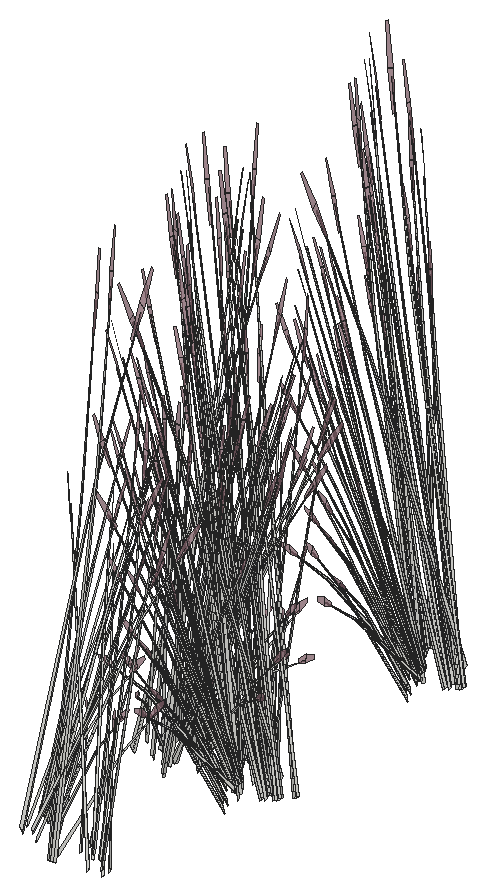
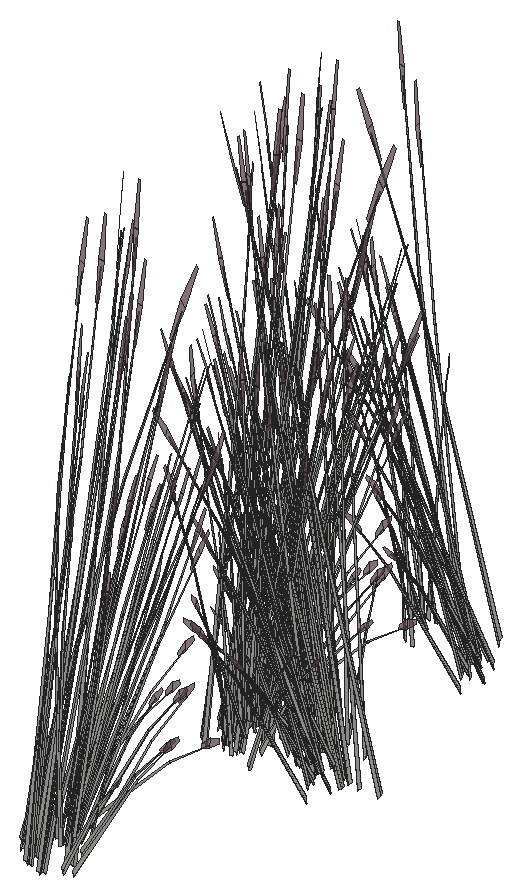
# SketchUp Ruby script. Lengths in inches.
U = 1.inch
M = Sketchup.active_model
def pt(a) = Geom::Point3d.new(a.map { |v| v * U })
def face(e, loops, mat)
  f = e.add_face(loops[0].map { |a| pt(a) })
  loops[1..].each { |l| e.add_face(l.map { |a| pt(a) }).erase! }
  f.material = f.back_material = mat if mat
  f
end
# faces: each face lists its corners as indices into pts; further lists are holes
def faces(e, pts, list, mat = nil) = list.each { |f| face(e, (f[0].is_a?(Array) ? f : [f]).map { |l| l.map { |i| pts[i] } }, mat) }
# xy, xz, yz: faces in a plane at the given z, y or x. An outline is a flat list of corners, or four numbers for a rectangle; further outlines are holes
def ring(l) = l.size == 4 ? [[l[0], l[1]], [l[2], l[1]], [l[2], l[3]], [l[0], l[3]]] : l.each_slice(2).to_a
def flat(e, list, mat, &to3) = list.each { |f| face(e, (f[0].is_a?(Array) ? f : [f]).map { |l| ring(l).map { |u, v| to3.(u, v) } }, mat) }
def xy(e, z, list, mat = nil) = flat(e, list, mat) { |x, y| [x, y, z] }
def xz(e, y, list, mat = nil) = flat(e, list, mat) { |x, z| [x, y, z] }
def yz(e, x, list, mat = nil) = flat(e, list, mat) { |y, z| [x, y, z] }
def lines(e, pts, list) = list.each { |a, b| e.add_line(pt(pts[a]), pt(pts[b])) }
# prism: a flat outline (further loops are holes) pulled along v
def prism(e, loops, v, mat = nil)
  f = face(e, loops, mat); d = Geom::Vector3d.new(v.map { |x| x * U })
  f.pushpull(f.normal.samedirection?(d) ? d.length : -d.length)
end
def box(e, o, s, mat = nil) = prism(e, [[o, [o[0] + s[0], o[1], o[2]], [o[0] + s[0], o[1] + s[1], o[2]], [o[0], o[1] + s[1], o[2]]]], [0, 0, s[2]], mat)
def at(x, y, z, deg = 0) = Geom::Transformation.translation(pt([x, y, z])) * Geom::Transformation.rotation(ORIGIN, Z_AXIS, deg.degrees)
def axes(o, x, y, z) = Geom::Transformation.new([*x, 0, *y, 0, *z, 0, *pt(o).to_a, 1])
def part(name) = M.definitions.add(name)
# library, detail: a bought-in or finely detailed component or shape, given as its bounding box
def library(name, o, s) = part(name).tap { |d| box(d.entities, o, s) }
def detail(e, o, s) = box(e.add_group.entities, o, s)
def put(e, d, t, mat = nil) = e.add_instance(d, t).tap { |i| i.material = mat if mat }
def group(e, t, mat = nil) = e.add_group.tap { |g| g.transformation = t; g.material = mat if mat }.entities
root = M.entities
M.materials.add("LightPink_Translucent").color = [144, 107, 117]
M.materials["LightPink_Translucent"].alpha = 0.75
c1 = part("blade")
p = [[2.15,0.21,22],[0,0.17,0],[0.09,0.45,0],[2.18,0.31,22],[2.29,0.31,22],[0.38,0.45,0],
  [2.48,0.24,33],[2.49,0.24,33],[2.48,0.22,33]]
faces(c1.entities,p,[[0,1,2,3],[4,5,2,3],[6,3,4,7],[8,0,3,6]])
c2 = part("seeds")
p = [[0.3,-0.1,1.38],[-0.01,-0.03,1.59],[-0.01,-0.03,0.03],[0.14,-0.07,-0.07],[0.29,-0.03,3],[0.15,0.01,3.11]]
faces(c2.entities,p,[[0,1,2,3],[1,0,4,5]],"LightPink_Translucent")
c3 = part("blade with seeds")
put(c3.entities,c1,at(0,0,0))
put(c3.entities,c2,axes([2.4,0.25,30.99],[1.5799,-0.05474,1.17369],[-0.12525,1.92788,0.29478],[-0.07173,-0.02425,1.56792]))
put(root,c3,axes([503.59,165.17,3.07],[0.14147,-0.21002,1.71376],[0.59349,0.43464,0.13857],[-0.26773,0.27089,0.73262]))
put(root,c3,axes([498.37,167.02,1.57],[0.95008,0,0],[0,0.68292,-0.51607],[0,0.15554,1.63711]))
put(root,c3,axes([503.76,166.35,3.72],[-0.5141,0.32171,-0.35414],[-0.48666,-0.36734,0.4572],[-0.07405,0.18664,0.87481]))
put(root,c3,axes([501.98,166.26,3.91],[-0.01889,0.12092,1.74944],[0.53598,0.42065,-0.27667],[-0.14032,0.19892,0.14031]))
put(root,c3,axes([497.58,168.53,3.72],[0.43232,0.38257,-0.35414],[-0.49364,0.36215,0.4572],[0.25081,0.0551,0.87481]))
put(root,c3,axes([497.36,168.68,3.92],[-0.03826,0.46465,0.0643],[-0.57772,-0.01274,0.50621],[0.2213,0.04862,0.77189]))
put(root,c3,axes([504.08,167.6,1.96],[-0.01966,-0.36332,1.1486],[0.49135,0.25914,0.84392],[-0.09663,0.17317,0.25299]))
put(root,c3,axes([497.42,168.53,3.93],[-0.56024,0.40262,0.48003],[-0.48318,-0.42758,0.3958],[0.26285,0.07427,0.9933]))
put(root,c3,axes([504.27,166.2,4.2],[0.54391,0.41056,-0.5672],[-0.57458,0.35956,-0.43934],[-0.08276,0.2086,1.08528]))
put(root,c3,axes([495.63,168.99,4.24],[-0.11735,-0.49217,0.35414],[0.67083,-0.12996,-0.4572],[0.18018,0.14104,0.87481]))
put(root,c3,axes([498.16,167.48,1.21],[0,0.61104,-0.49651],[-0.85008,0,0],[0,0.13917,1.57504]))
put(root,c3,axes([496.03,167.55,3.07],[-0.28223,-0.10528,1.71376],[0.58406,-0.44165,0.13857],[0.36402,0.19924,0.73262]))
put(root,c3,axes([496.08,166.16,3.67],[-0.65655,-0.31748,1.38283],[0.69326,-0.49431,0.59665],[0.21183,0.29789,1.33663]))
put(root,c3,axes([504.1,166.01,4.53],[-0.01977,0.56521,-0.7886],[-0.83252,-0.03796,0.09517],[-0.08786,0.23945,1.11556]))
put(root,c3,axes([501.92,167.5,3.9],[0.0862,-0.03689,1.77383],[0.71245,0.24539,-0.16761],[-0.01674,0.20431,0.31391]))
put(root,c3,axes([497.08,168.75,1.96],[-0.4278,-0.1757,1.1486],[0.5524,-0.17852,0.84392],[0.14899,0.15122,0.25299]))
put(root,c3,axes([495.57,169.25,4.23],[0.45276,-0.52302,-0.1216],[0.65568,0.30132,-0.67495],[0.22792,0.14777,1.02557]))
put(root,c3,axes([494.98,169.68,3.9],[0.00225,-0.07398,1.77383],[0.65113,-0.32638,-0.16761],[0.22617,0.1165,0.31391]))
put(root,c3,axes([497.2,169.4,0.6875],[0.05536,-0.08822,1.76342],[0.69692,-0.25981,-0.26939],[0.21129,0.13447,0.30037]))
put(root,c3,axes([496.11,168.99,3.875],[0.74975,-0.14525,-0.51099],[0.13115,0.55007,-0.3958],[0.20138,0.15763,0.97773]))
put(root,c3,axes([503.51,167.28,1.78],[0.23977,-0.09639,1.43002],[0.59198,0.29065,-0.30754],[-0.1762,0.25149,0.61141]))
put(root,c3,axes([497.14,169.55,1.86],[-0.48723,-0.01916,1.0506],[0.32177,-0.40701,0.58006],[0.19248,0.1446,0.8241]))
put(root,c3,axes([495.74,169.44,3.92],[-0.34533,0.38816,0.0643],[-0.49176,-0.22599,0.50621],[0.15898,0.12445,0.77189]))
put(root,c3,axes([495.89,169.33,3.93],[-0.75571,0.14023,0.48003],[-0.13115,-0.55007,0.3958],[0.17773,0.16212,0.9933]))
put(root,c3,axes([503.82,166.81,2.56],[0.01669,-0.31544,1.54345],[0.75083,0.16661,0.21329],[-0.06506,0.33618,0.72882]))
put(root,c3,axes([495.55,168.5625,1.78],[0.01341,-0.20255,1.43002],[0.64074,-0.22625,-0.30754],[0.1978,0.24243,0.61141]))
put(root,c3,axes([494.87,168.16,3.07],[-0.17368,-0.19618,1.71376],[0.80256,-0.16516,0.13857],[0.18139,0.30799,0.73262]))
put(root,c3,axes([504.63,183.77,3.07],[0.17368,0.19618,1.71376],[-0.80256,0.16516,0.13857],[-0.18139,-0.30799,0.73262]))
put(root,c3,axes([505.96,182.47,3.91],[-0.11621,-0.08567,1.74944],[-0.77555,0.05431,-0.27667],[-0.12378,-0.20491,0.14031]))
put(root,c3,axes([504.41,183.25,1.78],[-0.04601,0.19989,1.43002],[-0.67263,0.16733,-0.30754],[-0.15723,-0.25836,0.61141]))
put(root,c3,axes([505.16,182.1875,3.9],[-0.01417,0.07324,1.77383],[-0.6991,0.2658,-0.16761],[-0.20573,-0.13587,0.31391]))
put(root,c3,axes([505.01,183.49,4.29],[0.84639,-0.15705,0.53763],[0.14689,0.61608,0.4433],[-0.19906,-0.18157,1.11249]))
put(root,c3,axes([504.18,182.93,1.96],[0.39634,0.21267,1.1486],[-0.57721,0.12784,0.84392],[-0.1235,-0.16344,0.25299]))
put(root,c3,axes([505.14,184.06,4.17],[-0.64788,-0.29534,-0.71045],[0.46044,-0.51755,0.08574],[-0.23473,-0.17635,1.00501]))
put(root,c3,axes([504.91,183.66,3.72],[-0.11735,-0.49217,-0.35414],[0.67083,-0.12996,0.4572],[-0.18018,-0.14104,0.87481]))
put(root,c3,axes([505.2,183.62,3.92],[0.34533,-0.38816,0.0643],[0.49176,0.22599,0.50621],[-0.15898,-0.12445,0.77189]))
put(root,c3,axes([503.87,183.57,0.6875],[-0.0736,0.08049,1.76342],[-0.74378,0.17355,-0.26939],[-0.17968,-0.15788,0.30037]))
put(root,c3,axes([496.22,185,3.91],[-0.00733,-0.12161,1.74944],[-0.61946,-0.35147,-0.27667],[0.09577,-0.21306,0.14031]))
put(root,c3,axes([494.12,185.6,3.07],[-0.14147,0.21002,1.71376],[-0.59349,-0.43464,0.13857],[0.26773,-0.27089,0.73262]))
put(root,c3,axes([504.83,184.07,3.875],[-0.74975,0.14525,-0.51099],[-0.13115,-0.55007,-0.3958],[-0.20138,-0.15763,0.97773]))
put(root,c3,axes([505.36,183.58,4.62],[-0.50709,0.58578,-0.13619],[-0.73436,-0.33748,-0.75594],[-0.25527,-0.1655,1.14864]))
put(root,c3,axes([503.41,183.41,3.91],[-0.16348,-0.00431,1.74944],[-0.52047,0.43131,-0.27667],[-0.2777,-0.08813,0.14031]))
put(root,c3,axes([506.6875,187.4,2.52],[0.65659,0.2464,1.51261],[-0.64324,0.53082,0.59816],[-0.28812,-0.31461,1.26806]))
put(root,c3,axes([505.31,184.07,4.24],[0.11735,0.49217,0.35414],[-0.67083,0.12996,-0.4572],[-0.18018,-0.14104,0.87481]))
put(root,c3,axes([503.25,185.69,1.21],[0,-0.61104,-0.49651],[0.85008,0,0],[0,-0.13917,1.57504]))
put(root,c3,axes([503.29,184.39,4.29],[0.62747,-0.45094,0.53763],[0.54116,0.47889,0.4433],[-0.29439,-0.08318,1.11249]))
put(root,c3,axes([496.04,185.35,0.6875],[-0.11372,-0.04814,1.76342],[-0.29211,-0.53779,-0.26939],[0.19706,-0.14594,0.30037]))
put(root,c3,axes([495.4,185.67,3.93],[0.54105,0.41691,0.48003],[-0.57458,0.35956,0.3958],[0.0998,-0.1956,0.9933]))
put(root,c3,axes([503.58,184.38,3.92],[0.03826,-0.46465,0.0643],[0.57772,0.01274,0.50621],[-0.2213,-0.04862,0.77189]))
put(root,c3,axes([503.36,184.53,3.72],[-0.43232,-0.38257,-0.35414],[0.49364,-0.36215,0.4572],[-0.25081,-0.0551,0.87481]))
put(root,c3,axes([496.04,186.87,4.17],[0.39688,-0.48213,-0.71045],[0.69548,0.34264,0.08574],[0.23697,-0.17468,1.00501]))
put(root,c3,axes([503.4,183.88,1.32],[-0.21918,0.49894,-0.03893],[-0.6746,-0.15348,-0.17649],[-0.10242,-0.08161,0.58215]))
put(root,c3,axes([496.02,186.64,3.875],[-0.19519,-0.55794,-0.51099],[0.73919,-0.0976,-0.3958],[0.21183,-0.14986,0.97773]))
put(root,c3,axes([503.04,186.16,1.57],[-0.95008,0,0],[0,-0.68292,-0.51607],[0,-0.15554,1.63711]))
put(root,c3,axes([496.37,187.04,4.23],[-0.70283,-0.33692,-0.1216],[0.40491,-0.48793,-0.67495],[0.19857,-0.16961,1.02557]))
put(root,c3,axes([496.61,186.42,1.78],[-0.27143,-0.0181,1.43002],[-0.27808,-0.48551,-0.30754],[0.33346,-0.13735,0.61141]))
put(root,c3,axes([498.1,186.89,3.9],[-0.09924,-0.00464,1.77383],[-0.4121,-0.49725,-0.16761],[0.1655,-0.1635,0.31391]))
put(root,c3,axes([493.24,186.62,1.25],[0.51177,-0.45928,-0.62353],[0.63575,0.41646,-0.16365],[0.20507,-0.11457,1.37633]))
put(root,c3,axes([503.78,185.98,1.52],[-0.70674,0.51372,0.30756],[-0.70717,-0.50832,-0.36492],[-0.02468,-0.14589,1.64885]))
put(root,c3,axes([496.93,185.53,1.96],[-0.25308,0.31105,1.1486],[-0.21753,-0.4179,0.84392],[0.20902,-0.10472,0.25299]))
put(root,c3,axes([502.79,183.78,3.9],[0.05633,0.06098,1.77383],[-0.27155,0.54815,-0.16761],[-0.27501,0.00397,0.31391]))
put(root,c3,axes([505.69,187.05,1.63],[0.20138,-0.72405,-0.23429],[0.95485,0.12621,0.51271],[-0.16685,-0.09999,1.5644]))
put(root,c3,axes([496.57,186.7,3.72],[0.66138,-0.08733,-0.35414],[0.17464,0.49921,0.4572],[0.18953,-0.13408,0.87481]))
put(root,c3,axes([503.97,184.73,4.24],[0.43232,0.38257,0.35414],[-0.49364,0.36215,-0.4572],[-0.25081,-0.0551,0.87481]))
put(root,c3,axes([502.32,185.45,1.96],[0.48508,-0.04372,1.1486],[-0.3077,0.38525,0.84392],[-0.23971,-0.05779,0.25299]))
put(root,c3,axes([496.03,186.99,4.24],[-0.66138,0.08733,0.35414],[-0.17464,-0.49921,-0.4572],[0.18953,-0.13408,0.87481]))
put(root,c3,axes([503.85,184.49,4.23],[-0.04068,0.62141,-0.1216],[-0.77029,-0.01698,-0.67495],[-0.29667,-0.04317,1.02557]))
put(root,c3,axes([503.62,186.26,1.67],[0,0.61104,0.49651],[-0.85008,0,0],[0,-0.13917,1.57504]))
put(root,c3,axes([505.625,186.75,1.4],[-0.45644,-0.51287,-0.44739],[0.69137,-0.36116,0.21531],[-0.14771,-0.06346,1.43643]))
put(root,c3,axes([496.625,186.92,3.92],[0.52161,0.25698,0.0643],[-0.30368,0.36595,0.50621],[0.16723,-0.11831,0.77189]))
put(root,c3,axes([496.48,186.81,3.93],[0.18844,0.56237,0.48003],[-0.73919,0.0976,0.3958],[0.21785,-0.13226,0.9933]))
put(root,c3,axes([498.47,187.49,3.91],[0.10543,-0.09307,1.74944],[-0.13495,-0.57092,-0.27667],[0.26455,-0.10825,0.14031]))
put(root,c3,axes([505.22,186.95,1.25],[-0.79037,-0.10018,-0.62353],[0.16679,-0.61794,-0.16365],[-0.23587,-0.07488,1.37633]))
put(root,c3,axes([502.74,185.8,3.93],[0.21466,-0.55714,0.48003],[0.70573,0.19051,0.3958],[-0.27753,0.03348,0.9933]))
put(root,c3,axes([502.6875,185.65,3.92],[-0.27906,-0.41663,0.0643],[0.50888,-0.20393,0.50621],[-0.22432,0.04024,0.77189]))
put(root,c3,axes([504.375,187.89,1.22],[-0.17848,-0.53243,-0.30978],[0.70886,-0.15119,0.30978],[-0.1429,-0.0614,1.38974]))
put(root,c3,axes([496.4,188.36,4.23],[-0.38229,-0.5533,-0.1216],[0.6785,-0.2719,-0.67495],[0.28593,-0.073,1.02557]))
put(root,c3,axes([496.36,187.88,3.875],[0.20584,-0.55581,-0.51099],[0.70573,0.19051,-0.3958],[0.28414,-0.05097,0.97773]))
put(root,c3,axes([495.25,185.62,1.57],[0.47504,-0.61229,0],[0.79476,0.34146,-0.51607],[0.18101,0.07777,1.63711]))
put(root,c3,axes([504.18,188.12,1.21],[-0.7111,-0.30552,-0.49651],[0.42504,-0.54784,0],[-0.16196,-0.06958,1.57504]))
put(root,c3,axes([497.12,188.04,1.17],[-0.48937,0.07333,1.41583],[-0.07789,-0.58369,0.08104],[0.34275,-0.08835,0.80566]))
put(root,c3,axes([498.01,187.52,1.45],[-0.47106,-0.39072,-0.06488],[0.51591,-0.35801,-0.29416],[0.14618,-0.02521,0.97024]))
put(root,c3,axes([506.11,187.04,1.86],[-0.76714,0.40567,-0.29095],[-0.51013,-0.57321,-0.50002],[-0.18927,-0.05821,1.59708]))
put(root,c3,axes([496.23,188.08,4.17],[0.66765,-0.26986,-0.71045],[0.37208,0.55551,0.08574],[0.32259,-0.0631,1.00501]))
put(root,c3,axes([506.04,187.22,1.81],[-0.14658,0.54532,0.1448],[-0.71613,-0.09466,-0.41347],[-0.13033,-0.05599,1.26744]))
put(root,c3,axes([503.26,185.8,4.24],[0.63144,0.17046,0.35414],[-0.18417,0.49731,-0.4572],[-0.25423,0.0456,0.87481]))
put(root,c3,axes([496.13,188.1875,4.24],[-0.63144,-0.17046,0.35414],[0.18417,-0.49731,-0.4572],[0.25423,-0.0456,0.87481]))
put(root,c3,axes([491.81,186.7,0.79],[-0.74787,0.24464,1.28929],[-0.23804,-0.70192,0.50096],[0.45924,0.01168,1.46642]))
put(root,c3,axes([497.65,187.65,0.6875],[-0.03971,-0.09277,1.76342],[0.27541,-0.54264,-0.26939],[0.27782,-0.00781,0.30037]))
put(root,c3,axes([506.97,187.23,1.66],[-0.74193,-0.49181,-0.25192],[0.6243,-0.55226,0.5513],[-0.19979,0.05753,1.68216]))
put(root,c3,axes([505.02,188.17,1.67],[0.7111,0.30552,0.49651],[-0.42504,0.54784,0],[-0.16196,-0.06958,1.57504]))
put(root,c3,axes([493.75,187.0625,1.86],[0.76714,-0.40567,-0.29095],[0.51013,0.57321,-0.50002],[0.18927,0.05821,1.59708]))
put(root,c3,axes([496.8,188.13,3.72],[0.63144,0.17046,-0.35414],[-0.18417,0.49731,0.4572],[0.25423,-0.0456,0.87481]))
put(root,c3,axes([495.68,185.99,1.21],[0.7111,0.30552,-0.49651],[-0.42504,0.54784,0],[0.16196,0.06958,1.57504]))
put(root,c3,axes([503,185.64,4.23],[0.38229,0.5533,-0.1216],[-0.6785,0.2719,-0.67495],[-0.28593,0.073,1.02557]))
put(root,c3,axes([504.61,188.49,1.57],[-0.47504,0.61229,0],[-0.79476,-0.34146,-0.51607],[-0.18101,-0.07777,1.63711]))
put(root,c3,axes([495.08,187.52,3.07],[-0.31515,0.01384,1.71376],[0.20907,-0.5998,0.13857],[0.44912,0.0371,0.73262]))
put(root,c3,axes([495.48,186.21,1.22],[0.17848,0.53243,-0.30978],[-0.70886,0.15119,0.30978],[0.1429,0.0614,1.38974]))
put(root,c3,axes([506.6,187.12,1.4],[-0.82508,0.03772,-0.44739],[-0.07462,-0.62614,0.21531],[-0.14771,0.06346,1.43643]))
put(root,c3,axes([496.7,188.34,3.92],[0.27906,0.41663,0.0643],[-0.50888,0.20393,0.50621],[0.22432,-0.04024,0.77189]))
put(root,c3,axes([496.65,188.19,3.93],[-0.21466,0.55714,0.48003],[-0.70573,-0.19051,0.3958],[0.27753,-0.03348,0.9933]))
put(root,c3,axes([507.51,188.57,1.39],[-0.46912,-0.61443,-0.05142],[0.79476,-0.34146,0.51607],[-0.19584,0.0585,1.6363]))
put(root,c3,axes([502.91,187.18,3.93],[-0.18844,-0.56237,0.48003],[0.73919,-0.0976,0.3958],[-0.21785,0.13226,0.9933]))
put(root,c3,axes([502.77,187.08,3.92],[-0.52161,-0.25698,0.0643],[0.30368,-0.36595,0.50621],[-0.16723,0.11831,0.77189]))
put(root,c3,axes([494.64,187.16,1.25],[0.79037,0.10018,-0.62353],[-0.16679,0.61794,-0.16365],[0.23587,0.07488,1.37633]))
put(root,c3,axes([498.14,188.23,1.96],[-0.46945,0.10088,1.1486],[0.22097,-0.4169,0.84392],[0.24904,0.02853,0.25299]))
put(root,c3,axes([497.92,190,3.9],[-0.0687,-0.05349,1.77383],[0.15029,-0.57341,-0.16761],[0.27062,-0.03664,0.31391]))
put(root,c3,axes([497.32,189.52,3.12],[-0.14542,-0.51365,-0.03492],[0.68734,-0.11809,-0.15832],[0.14353,0.03256,0.52218]))
put(root,c3,axes([495.54,189.5,4.23],[0.04068,-0.62141,-0.1216],[0.77029,0.01698,-0.67495],[0.29667,0.04317,1.02557]))
put(root,c3,axes([503.37,187,4.24],[0.66138,-0.08733,0.35414],[0.17464,0.49921,-0.4572],[-0.18953,0.13408,0.87481]))
put(root,c3,axes([501.63,188.49,1.96],[0.31665,-0.27694,1.1486],[0.12495,0.43841,0.84392],[-0.22883,0.0785,0.25299]))
put(root,c3,axes([495.42,189.26,4.24],[-0.43232,-0.38257,0.35414],[0.49364,-0.36215,-0.4572],[0.25081,0.0551,0.87481]))
put(root,c3,axes([502.83,187.29,3.72],[-0.66138,0.08733,-0.35414],[-0.17464,-0.49921,0.4572],[-0.18953,0.13408,0.87481]))
put(root,c3,axes([501.87,188.41,4.84],[0.67048,0.16311,-0.06488],[-0.20625,0.50201,-0.29416],[-0.10966,0.07622,0.97024]))
put(root,c3,axes([506.62,187.48,1.25],[-0.51177,0.45928,-0.62353],[-0.63575,-0.41646,-0.16365],[-0.20507,0.11457,1.37633]))
put(root,c3,axes([496.21,189.13,3.91],[0.16299,-0.01033,1.74944],[0.44707,-0.47471,-0.27667],[0.28992,0.06266,0.14031]))
put(root,c3,axes([507.46,188.74,1.21],[-0.7111,0.30552,-0.49651],[-0.42504,-0.54784,0],[-0.16196,0.06958,1.57504]))
put(root,c3,axes([495.58,189.21,4.17],[0.75952,0.01471,-0.71045],[-0.05101,0.61953,0.08574],[0.32177,0.06538,1.00501]))
put(root,c3,axes([503.02,186.95,4.23],[0.70283,0.33692,-0.1216],[-0.40491,0.48793,-0.67495],[-0.19857,0.16961,1.02557]))
put(root,c3,axes([503.97,186.8,3.07],[0.18977,-0.18775,1.71376],[0.47917,0.50677,0.13857],[-0.32866,0.23079,0.73262]))
put(root,c3,axes([503.37,187.35,3.875],[0.19519,0.55794,-0.51099],[-0.73919,0.0976,-0.3958],[-0.21183,0.14986,0.97773]))
put(root,c3,axes([496.82,187.95,1.57],[0.95008,0,0],[0,0.68292,-0.51607],[0,0.15554,1.63711]))
put(root,c3,axes([496.03,189.46,3.72],[0.43232,0.38257,-0.35414],[-0.49364,0.36215,0.4572],[0.25081,0.0551,0.87481]))
put(root,c3,axes([503.79,188.28,3.92],[-0.62439,-0.02847,0.0643],[0.01712,-0.42991,0.50621],[-0.06534,0.16468,0.77189]))
put(root,c3,axes([495.8125,189.61,3.92],[-0.03826,0.46465,0.0643],[-0.57772,-0.01274,0.50621],[0.2213,0.04862,0.77189]))
put(root,c3,axes([502.47,188.77,0.6875],[0.10192,0.06105,1.76342],[0.17281,0.56562,-0.26939],[-0.22588,0.12062,0.30037]))
put(root,c3,axes([503.99,188.32,3.93],[-0.54105,-0.41691,0.48003],[0.57458,-0.35956,0.3958],[-0.0998,0.1956,0.9933]))
put(root,c3,axes([495.86,189.46,3.93],[-0.56024,0.40262,0.48003],[-0.48318,-0.42758,0.3958],[0.26285,0.07427,0.9933]))
put(root,c3,axes([494.48,188.48,3.07],[-0.28223,-0.10528,1.71376],[0.58406,-0.44165,0.13857],[0.36402,0.19924,0.73262]))
put(root,c3,axes([503.83,187.26,3.07],[0.14147,-0.21002,1.71376],[0.59349,0.43464,0.13857],[-0.26773,0.27089,0.73262]))
put(root,c3,axes([495.53,189.68,1.96],[-0.4278,-0.1757,1.1486],[0.5524,-0.17852,0.84392],[0.14899,0.15122,0.25299]))
put(root,c3,axes([494.02,190.18,4.23],[0.45276,-0.52302,-0.1216],[0.65568,0.30132,-0.67495],[0.22792,0.14777,1.02557]))
put(root,c3,axes([503.99,188.45,3.72],[-0.5141,0.32171,-0.35414],[-0.48666,-0.36734,0.4572],[-0.07405,0.18664,0.87481]))
put(root,c3,axes([502.22,188.35,3.91],[-0.01889,0.12092,1.74944],[0.53598,0.42065,-0.27667],[-0.14032,0.19892,0.14031]))
put(root,c3,axes([504.32,189.7,1.96],[-0.01966,-0.36332,1.1486],[0.49135,0.25914,0.84392],[-0.09663,0.17317,0.25299]))
put(root,c3,axes([495.65,190.33,0.6875],[0.05536,-0.08822,1.76342],[0.69692,-0.25981,-0.26939],[0.21129,0.13447,0.30037]))
put(root,c3,axes([494.56,189.92,3.875],[0.74975,-0.14525,-0.51099],[0.13115,0.55007,-0.3958],[0.20138,0.15763,0.97773]))
put(root,c3,axes([495.59,190.48,1.86],[-0.48723,-0.01916,1.0506],[0.32177,-0.40701,0.58006],[0.19248,0.1446,0.8241]))
put(root,c3,axes([504.33,188.11,4.53],[-0.01977,0.56521,-0.7886],[-0.83252,-0.03796,0.09517],[-0.08786,0.23945,1.11556]))
put(root,c3,axes([502.16,189.59,3.9],[0.0862,-0.03689,1.77383],[0.71245,0.24539,-0.16761],[-0.01674,0.20431,0.31391]))
put(root,c3,axes([494,189.49,1.78],[0.01341,-0.20255,1.43002],[0.64074,-0.22625,-0.30754],[0.1978,0.24243,0.61141]))
put(root,c3,axes([503.75,189.375,1.78],[0.23977,-0.09639,1.43002],[0.59198,0.29065,-0.30754],[-0.1762,0.25149,0.61141]))
put(root,c3,axes([504.06,188.9,2.56],[0.01669,-0.31544,1.54345],[0.75083,0.16661,0.21329],[-0.06506,0.33618,0.72882]))
put(root,c3,axes([504.76,208.02,3.07],[0.17368,0.19618,1.71376],[-0.80256,0.16516,0.13857],[-0.18139,-0.30799,0.73262]))
put(root,c3,axes([506.09,206.72,3.91],[-0.11621,-0.08567,1.74944],[-0.77555,0.05431,-0.27667],[-0.12378,-0.20491,0.14031]))
put(root,c3,axes([504.54,207.5,1.78],[-0.04601,0.19989,1.43002],[-0.67263,0.16733,-0.30754],[-0.15723,-0.25836,0.61141]))
put(root,c3,axes([505.29,206.4375,3.9],[-0.01417,0.07324,1.77383],[-0.6991,0.2658,-0.16761],[-0.20573,-0.13587,0.31391]))
put(root,c3,axes([505.14,207.74,4.29],[0.84639,-0.15705,0.53763],[0.14689,0.61608,0.4433],[-0.19906,-0.18157,1.11249]))
put(root,c3,axes([504.3125,207.18,1.96],[0.39634,0.21267,1.1486],[-0.57721,0.12784,0.84392],[-0.1235,-0.16344,0.25299]))
put(root,c3,axes([505.27,208.31,4.17],[-0.64788,-0.29534,-0.71045],[0.46044,-0.51755,0.08574],[-0.23473,-0.17635,1.00501]))
put(root,c3,axes([505.04,207.92,3.72],[-0.11735,-0.49217,-0.35414],[0.67083,-0.12996,0.4572],[-0.18018,-0.14104,0.87481]))
put(root,c3,axes([505.33,207.87,3.92],[0.34533,-0.38816,0.0643],[0.49176,0.22599,0.50621],[-0.15898,-0.12445,0.77189]))
put(root,c3,axes([504,207.82,0.6875],[-0.0736,0.08049,1.76342],[-0.74378,0.17355,-0.26939],[-0.17968,-0.15788,0.30037]))
put(root,c3,axes([504.96,208.32,3.875],[-0.74975,0.14525,-0.51099],[-0.13115,-0.55007,-0.3958],[-0.20138,-0.15763,0.97773]))
put(root,c3,axes([505.49,207.83,4.62],[-0.50709,0.58578,-0.13619],[-0.73436,-0.33748,-0.75594],[-0.25527,-0.1655,1.14864]))
put(root,c3,axes([503.54,207.66,3.91],[-0.16348,-0.00431,1.74944],[-0.52047,0.43131,-0.27667],[-0.2777,-0.08813,0.14031]))
put(root,c3,axes([506.82,211.65,2.52],[0.65659,0.2464,1.51261],[-0.64324,0.53082,0.59816],[-0.28812,-0.31461,1.26806]))
put(root,c3,axes([505.44,208.32,4.24],[0.11735,0.49217,0.35414],[-0.67083,0.12996,-0.4572],[-0.18018,-0.14104,0.87481]))
put(root,c3,axes([503.42,208.64,4.29],[0.62747,-0.45094,0.53763],[0.54116,0.47889,0.4433],[-0.29439,-0.08318,1.11249]))
put(root,c3,axes([503.71,208.64,3.92],[0.03826,-0.46465,0.0643],[0.57772,0.01274,0.50621],[-0.2213,-0.04862,0.77189]))
put(root,c3,axes([503.49,208.78,3.72],[-0.43232,-0.38257,-0.35414],[0.49364,-0.36215,0.4572],[-0.25081,-0.0551,0.87481]))
put(root,c3,axes([503.53,208.13,1.32],[-0.21918,0.49894,-0.03893],[-0.6746,-0.15348,-0.17649],[-0.10242,-0.08161,0.58215]))
put(root,c3,axes([503.17,210.41,1.57],[-0.95008,0,0],[0,-0.68292,-0.51607],[0,-0.15554,1.63711]))
put(root,c3,axes([503.91,210.23,1.52],[-0.70674,0.51372,0.30756],[-0.70717,-0.50832,-0.36492],[-0.02468,-0.14589,1.64885]))
put(root,c3,axes([502.92,208.03,3.9],[0.05633,0.06098,1.77383],[-0.27155,0.54815,-0.16761],[-0.27501,0.00397,0.31391]))
put(root,c3,axes([505.82,211.3,1.63],[0.20138,-0.72405,-0.23429],[0.95485,0.12621,0.51271],[-0.16685,-0.09999,1.5644]))
put(root,c3,axes([503.69,209.16,3.875],[-0.55171,0.40476,-0.51099],[-0.48318,-0.42758,-0.3958],[-0.28031,-0.06159,0.97773]))
put(root,c3,axes([504.1,208.98,4.24],[0.43232,0.38257,0.35414],[-0.49364,0.36215,-0.4572],[-0.25081,-0.0551,0.87481]))
put(root,c3,axes([502.45,209.7,1.96],[0.48508,-0.04372,1.1486],[-0.3077,0.38525,0.84392],[-0.23971,-0.05779,0.25299]))
put(root,c3,axes([503.98,208.74,4.23],[-0.04068,0.62141,-0.1216],[-0.77029,-0.01698,-0.67495],[-0.29667,-0.04317,1.02557]))
put(root,c3,axes([505.76,211.01,1.4],[-0.45644,-0.51287,-0.44739],[0.69137,-0.36116,0.21531],[-0.14771,-0.06346,1.43643]))
put(root,c3,axes([505.35,211.2,1.25],[-0.79037,-0.10018,-0.62353],[0.16679,-0.61794,-0.16365],[-0.23587,-0.07488,1.37633]))
put(root,c3,axes([502.875,210.05,3.93],[0.21466,-0.55714,0.48003],[0.70573,0.19051,0.3958],[-0.27753,0.03348,0.9933]))
put(root,c3,axes([502.82,209.9,3.92],[-0.27906,-0.41663,0.0643],[0.50888,-0.20393,0.50621],[-0.22432,0.04024,0.77189]))
put(root,c3,axes([502.81,210.33,0.6875],[0.01927,0.0963,1.76342],[-0.38846,0.5029,-0.26939],[-0.27592,-0.02535,0.30037]))
put(root,c3,axes([504.51,212.14,1.22],[-0.17848,-0.53243,-0.30978],[0.70886,-0.15119,0.30978],[-0.1429,-0.0614,1.38974]))
put(root,c3,axes([504.31,212.37,1.21],[-0.7111,-0.30552,-0.49651],[0.42504,-0.54784,0],[-0.16196,-0.06958,1.57504]))
put(root,c3,axes([506.24,211.29,1.86],[-0.76714,0.40567,-0.29095],[-0.51013,-0.57321,-0.50002],[-0.18927,-0.05821,1.59708]))
put(root,c3,axes([506.17,211.47,1.81],[-0.14658,0.54532,0.1448],[-0.71613,-0.09466,-0.41347],[-0.13033,-0.05599,1.26744]))
put(root,c3,axes([503.39,210.06,4.24],[0.63144,0.17046,0.35414],[-0.18417,0.49731,-0.4572],[-0.25423,0.0456,0.87481]))
put(root,c3,axes([507.1,211.48,1.66],[-0.74193,-0.49181,-0.25192],[0.6243,-0.55226,0.5513],[-0.19979,0.05753,1.68216]))
put(root,c3,axes([505.15,212.42,1.67],[0.7111,0.30552,0.49651],[-0.42504,0.54784,0],[-0.16196,-0.06958,1.57504]))
put(root,c3,axes([503.125,209.89,4.23],[0.38229,0.5533,-0.1216],[-0.6785,0.2719,-0.67495],[-0.28593,0.073,1.02557]))
put(root,c3,axes([504.74,212.74,1.57],[-0.47504,0.61229,0],[-0.79476,-0.34146,-0.51607],[-0.18101,-0.07777,1.63711]))
put(root,c3,axes([506.73,211.375,1.4],[-0.82508,0.03772,-0.44739],[-0.07462,-0.62614,0.21531],[-0.14771,0.06346,1.43643]))
put(root,c3,axes([503.04,211.4375,3.93],[-0.18844,-0.56237,0.48003],[0.73919,-0.0976,0.3958],[-0.21785,0.13226,0.9933]))
put(root,c3,axes([502.9,211.33,3.92],[-0.52161,-0.25698,0.0643],[0.30368,-0.36595,0.50621],[-0.16723,0.11831,0.77189]))
put(root,c3,axes([503.5,211.25,4.24],[0.66138,-0.08733,0.35414],[0.17464,0.49921,-0.4572],[-0.18953,0.13408,0.87481]))
put(root,c3,axes([501.76,212.74,1.96],[0.31665,-0.27694,1.1486],[0.12495,0.43841,0.84392],[-0.22883,0.0785,0.25299]))
put(root,c3,axes([502.96,211.54,3.72],[-0.66138,0.08733,-0.35414],[-0.17464,-0.49921,0.4572],[-0.18953,0.13408,0.87481]))
put(root,c3,axes([502,212.67,4.84],[0.67048,0.16311,-0.06488],[-0.20625,0.50201,-0.29416],[-0.10966,0.07622,0.97024]))
put(root,c3,axes([506.75,211.74,1.25],[-0.51177,0.45928,-0.62353],[-0.63575,-0.41646,-0.16365],[-0.20507,0.11457,1.37633]))
